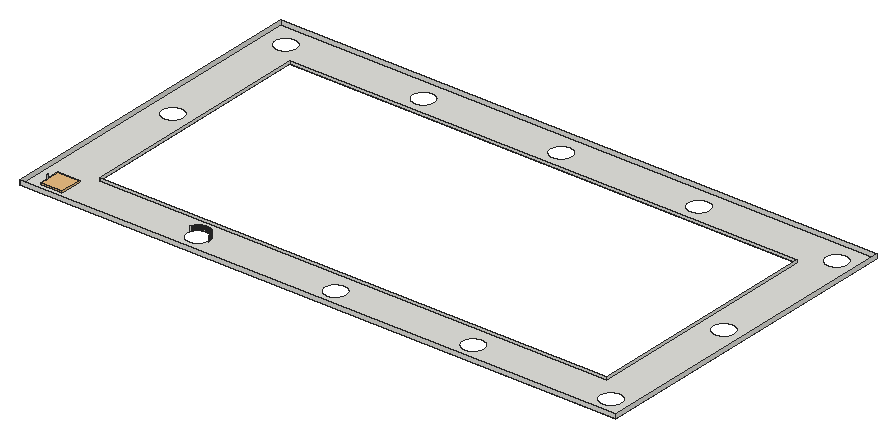
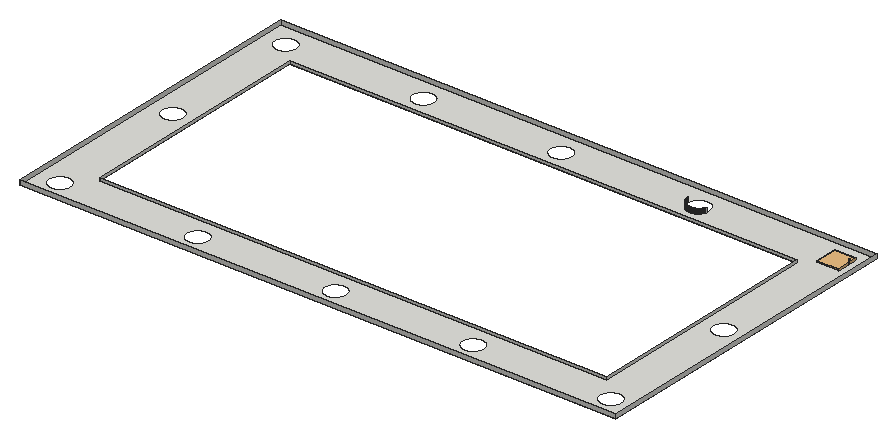
# SketchUp Ruby script. Lengths in inches.
U = 1.inch
M = Sketchup.active_model
def pt(a) = Geom::Point3d.new(a.map { |v| v * U })
def face(e, loops, mat)
  f = e.add_face(loops[0].map { |a| pt(a) })
  loops[1..].each { |l| e.add_face(l.map { |a| pt(a) }).erase! }
  f.material = f.back_material = mat if mat
  f
end
# faces: each face lists its corners as indices into pts; further lists are holes
def faces(e, pts, list, mat = nil) = list.each { |f| face(e, (f[0].is_a?(Array) ? f : [f]).map { |l| l.map { |i| pts[i] } }, mat) }
# xy, xz, yz: faces in a plane at the given z, y or x. An outline is a flat list of corners, or four numbers for a rectangle; further outlines are holes
def ring(l) = l.size == 4 ? [[l[0], l[1]], [l[2], l[1]], [l[2], l[3]], [l[0], l[3]]] : l.each_slice(2).to_a
def flat(e, list, mat, &to3) = list.each { |f| face(e, (f[0].is_a?(Array) ? f : [f]).map { |l| ring(l).map { |u, v| to3.(u, v) } }, mat) }
def xy(e, z, list, mat = nil) = flat(e, list, mat) { |x, y| [x, y, z] }
def xz(e, y, list, mat = nil) = flat(e, list, mat) { |x, z| [x, y, z] }
def yz(e, x, list, mat = nil) = flat(e, list, mat) { |y, z| [x, y, z] }
def lines(e, pts, list) = list.each { |a, b| e.add_line(pt(pts[a]), pt(pts[b])) }
# prism: a flat outline (further loops are holes) pulled along v
def prism(e, loops, v, mat = nil)
  f = face(e, loops, mat); d = Geom::Vector3d.new(v.map { |x| x * U })
  f.pushpull(f.normal.samedirection?(d) ? d.length : -d.length)
end
def box(e, o, s, mat = nil) = prism(e, [[o, [o[0] + s[0], o[1], o[2]], [o[0] + s[0], o[1] + s[1], o[2]], [o[0], o[1] + s[1], o[2]]]], [0, 0, s[2]], mat)
def at(x, y, z, deg = 0) = Geom::Transformation.translation(pt([x, y, z])) * Geom::Transformation.rotation(ORIGIN, Z_AXIS, deg.degrees)
def axes(o, x, y, z) = Geom::Transformation.new([*x, 0, *y, 0, *z, 0, *pt(o).to_a, 1])
def part(name) = M.definitions.add(name)
# library, detail: a bought-in or finely detailed component or shape, given as its bounding box
def library(name, o, s) = part(name).tap { |d| box(d.entities, o, s) }
def detail(e, o, s) = box(e.add_group.entities, o, s)
def put(e, d, t, mat = nil) = e.add_instance(d, t).tap { |i| i.material = mat if mat }
def group(e, t, mat = nil) = e.add_group.tap { |g| g.transformation = t; g.material = mat if mat }.entities
root = M.entities
c1 = library("plafonjera p5",[102.27,51.27,12.6],[3.93,3.93,0.39])
xy(root,231.53,[[[57.99,28,382.75,206],[81.99,52,358.75,182],[370.5625,188,370.9375,188,371.31,188.03,371.6875,188.07,372.06,188.14,372.42,188.24,372.78,188.35,373.13,188.49,373.47,188.65,373.8,188.84,374.12,189.04,374.43,189.26,374.72,189.5,374.99,189.76,375.25,190.03,375.49,190.32,375.71,190.63,375.91,190.95,376.1,191.28,376.26,191.62,376.4,191.97,376.51,192.33,376.61,192.69,376.68,193.0625,376.72,193.44,376.75,193.8125,376.75,194.1875,376.72,194.56,376.68,194.9375,376.61,195.31,376.51,195.67,376.4,196.03,376.26,196.38,376.1,196.72,375.91,197.05,375.71,197.37,375.49,197.68,375.25,197.97,374.99,198.24,374.72,198.5,374.43,198.74,374.12,198.96,373.8,199.16,373.47,199.35,373.13,199.51,372.78,199.65,372.42,199.76,372.06,199.86,371.6875,199.93,371.31,199.97,370.9375,200,370.5625,200,370.19,199.97,369.8125,199.93,369.44,199.86,369.08,199.76,368.72,199.65,368.37,199.51,368.03,199.35,367.7,199.16,367.38,198.96,367.07,198.74,366.78,198.5,366.51,198.24,366.25,197.97,366.01,197.68,365.79,197.37,365.59,197.05,365.4,196.72,365.24,196.38,365.1,196.03,364.99,195.67,364.89,195.31,364.82,194.9375,364.78,194.56,364.75,194.1875,364.75,193.8125,364.78,193.44,364.82,193.0625,364.89,192.69,364.99,192.33,365.1,191.97,365.24,191.62,365.4,191.28,365.59,190.95,365.79,190.63,366.01,190.32,366.25,190.03,366.51,189.76,366.78,189.5,367.07,189.26,367.38,189.04,367.7,188.84,368.03,188.65,368.37,188.49,368.72,188.35,369.08,188.24,369.44,188.14,369.8125,188.07,370.19,188.03],[220.18,188,220.56,188,220.94,188.03,221.31,188.07,221.68,188.14,222.04,188.24,222.4,188.35,222.75,188.49,223.09,188.65,223.43,188.84,223.74,189.04,224.05,189.26,224.34,189.5,224.61,189.76,224.87,190.03,225.11,190.32,225.33,190.63,225.54,190.95,225.72,191.28,225.88,191.62,226.02,191.97,226.13,192.33,226.23,192.69,226.3,193.0625,226.34,193.44,226.37,193.8125,226.37,194.1875,226.34,194.56,226.3,194.9375,226.23,195.31,226.13,195.67,226.02,196.03,225.88,196.38,225.72,196.72,225.54,197.05,225.33,197.37,225.11,197.68,224.87,197.97,224.61,198.24,224.34,198.5,224.05,198.74,223.74,198.96,223.43,199.16,223.09,199.35,222.75,199.51,222.4,199.65,222.04,199.76,221.68,199.86,221.31,199.93,220.94,199.97,220.56,200,220.18,200,219.81,199.97,219.43,199.93,219.0625,199.86,218.7,199.76,218.34,199.65,217.99,199.51,217.65,199.35,217.32,199.16,217,198.96,216.69,198.74,216.4,198.5,216.13,198.24,215.87,197.97,215.63,197.68,215.41,197.37,215.21,197.05,215.02,196.72,214.86,196.38,214.73,196.03,214.61,195.67,214.52,195.31,214.44,194.9375,214.4,194.56,214.375,194.1875,214.375,193.8125,214.4,193.44,214.44,193.0625,214.52,192.69,214.61,192.33,214.73,191.97,214.86,191.62,215.02,191.28,215.21,190.95,215.41,190.63,215.63,190.32,215.87,190.03,216.13,189.76,216.4,189.5,216.69,189.26,217,189.04,217.32,188.84,217.65,188.65,217.99,188.49,218.34,188.35,218.7,188.24,219.0625,188.14,219.43,188.07,219.81,188.03],[295.37,188,295.75,188,296.125,188.03,296.5,188.07,296.87,188.14,297.23,188.24,297.59,188.35,297.94,188.49,298.28,188.65,298.61,188.84,298.93,189.04,299.24,189.26,299.53,189.5,299.8,189.76,300.0625,190.03,300.3,190.32,300.52,190.63,300.72,190.95,300.91,191.28,301.07,191.62,301.21,191.97,301.32,192.33,301.42,192.69,301.49,193.0625,301.53,193.44,301.56,193.8125,301.56,194.1875,301.53,194.56,301.49,194.9375,301.42,195.31,301.32,195.67,301.21,196.03,301.07,196.38,300.91,196.72,300.72,197.05,300.52,197.37,300.3,197.68,300.0625,197.97,299.8,198.24,299.53,198.5,299.24,198.74,298.93,198.96,298.61,199.16,298.28,199.35,297.94,199.51,297.59,199.65,297.23,199.76,296.87,199.86,296.5,199.93,296.125,199.97,295.75,200,295.37,200,295,199.97,294.62,199.93,294.25,199.86,293.89,199.76,293.53,199.65,293.18,199.51,292.84,199.35,292.51,199.16,292.1875,198.96,291.88,198.74,291.59,198.5,291.32,198.24,291.06,197.97,290.82,197.68,290.6,197.37,290.4,197.05,290.21,196.72,290.05,196.38,289.92,196.03,289.8,195.67,289.7,195.31,289.63,194.9375,289.59,194.56,289.5625,194.1875,289.5625,193.8125,289.59,193.44,289.63,193.0625,289.7,192.69,289.8,192.33,289.92,191.97,290.05,191.62,290.21,191.28,290.4,190.95,290.6,190.63,290.82,190.32,291.06,190.03,291.32,189.76,291.59,189.5,291.88,189.26,292.1875,189.04,292.51,188.84,292.84,188.65,293.18,188.49,293.53,188.35,293.89,188.24,294.25,188.14,294.62,188.07,295,188.03],[370.5625,111,370.9375,111,371.31,111.03,371.6875,111.07,372.06,111.14,372.42,111.24,372.78,111.35,373.13,111.49,373.47,111.65,373.8,111.84,374.12,112.04,374.43,112.26,374.72,112.5,374.99,112.76,375.25,113.03,375.49,113.32,375.71,113.63,375.91,113.95,376.1,114.28,376.26,114.62,376.4,114.97,376.51,115.33,376.61,115.69,376.68,116.0625,376.72,116.44,376.75,116.8125,376.75,117.1875,376.72,117.56,376.68,117.9375,376.61,118.31,376.51,118.67,376.4,119.03,376.26,119.38,376.1,119.72,375.91,120.05,375.71,120.37,375.49,120.68,375.25,120.97,374.99,121.24,374.72,121.5,374.43,121.74,374.12,121.96,373.8,122.16,373.47,122.35,373.13,122.51,372.78,122.65,372.42,122.76,372.06,122.86,371.6875,122.93,371.31,122.97,370.9375,123,370.5625,123,370.19,122.97,369.8125,122.93,369.44,122.86,369.08,122.76,368.72,122.65,368.37,122.51,368.03,122.35,367.7,122.16,367.38,121.96,367.07,121.74,366.78,121.5,366.51,121.24,366.25,120.97,366.01,120.68,365.79,120.37,365.59,120.05,365.4,119.72,365.24,119.38,365.1,119.03,364.99,118.67,364.89,118.31,364.82,117.9375,364.78,117.56,364.75,117.1875,364.75,116.8125,364.78,116.44,364.82,116.0625,364.89,115.69,364.99,115.33,365.1,114.97,365.24,114.62,365.4,114.28,365.59,113.95,365.79,113.63,366.01,113.32,366.25,113.03,366.51,112.76,366.78,112.5,367.07,112.26,367.38,112.04,367.7,111.84,368.03,111.65,368.37,111.49,368.72,111.35,369.08,111.24,369.44,111.14,369.8125,111.07,370.19,111.03],[69.8,34,70.18,34,70.56,34.03,70.93,34.07,71.3,34.14,71.67,34.24,72.02,34.35,72.375,34.49,72.72,34.65,73.05,34.84,73.36,35.04,73.67,35.26,73.96,35.5,74.23,35.76,74.49,36.03,74.73,36.32,74.95,36.63,75.16,36.95,75.34,37.28,75.5,37.62,75.64,37.97,75.75,38.33,75.85,38.69,75.92,39.0625,75.96,39.44,75.99,39.8125,75.99,40.1875,75.96,40.56,75.92,40.9375,75.85,41.31,75.75,41.67,75.64,42.03,75.5,42.38,75.34,42.72,75.16,43.05,74.95,43.37,74.73,43.68,74.49,43.97,74.23,44.24,73.96,44.5,73.67,44.74,73.36,44.96,73.05,45.16,72.72,45.35,72.375,45.51,72.02,45.65,71.67,45.76,71.3,45.86,70.93,45.93,70.56,45.97,70.18,46,69.8,46,69.43,45.97,69.05,45.93,68.68,45.86,68.32,45.76,67.96,45.65,67.61,45.51,67.27,45.35,66.9375,45.16,66.62,44.96,66.3125,44.74,66.02,44.5,65.75,44.24,65.49,43.97,65.25,43.68,65.03,43.37,64.83,43.05,64.65,42.72,64.48,42.38,64.35,42.03,64.23,41.67,64.14,41.31,64.07,40.9375,64.02,40.56,63.99,40.1875,63.99,39.8125,64.02,39.44,64.07,39.0625,64.14,38.69,64.23,38.33,64.35,37.97,64.48,37.62,64.65,37.28,64.83,36.95,65.03,36.63,65.25,36.32,65.49,36.03,65.75,35.76,66.02,35.5,66.3125,35.26,66.62,35.04,66.9375,34.84,67.27,34.65,67.61,34.49,67.96,34.35,68.32,34.24,68.68,34.14,69.05,34.07,69.43,34.03],[69.8,111,70.18,111,70.56,111.03,70.93,111.07,71.3,111.14,71.67,111.24,72.02,111.35,72.375,111.49,72.72,111.65,73.05,111.84,73.36,112.04,73.67,112.26,73.96,112.5,74.23,112.76,74.49,113.03,74.73,113.32,74.95,113.63,75.16,113.95,75.34,114.28,75.5,114.62,75.64,114.97,75.75,115.33,75.85,115.69,75.92,116.0625,75.96,116.44,75.99,116.8125,75.99,117.1875,75.96,117.56,75.92,117.9375,75.85,118.31,75.75,118.67,75.64,119.03,75.5,119.38,75.34,119.72,75.16,120.05,74.95,120.37,74.73,120.68,74.49,120.97,74.23,121.24,73.96,121.5,73.67,121.74,73.36,121.96,73.05,122.16,72.72,122.35,72.375,122.51,72.02,122.65,71.67,122.76,71.3,122.86,70.93,122.93,70.56,122.97,70.18,123,69.8,123,69.43,122.97,69.05,122.93,68.68,122.86,68.32,122.76,67.96,122.65,67.61,122.51,67.27,122.35,66.9375,122.16,66.62,121.96,66.3125,121.74,66.02,121.5,65.75,121.24,65.49,120.97,65.25,120.68,65.03,120.37,64.83,120.05,64.65,119.72,64.48,119.38,64.35,119.03,64.23,118.67,64.14,118.31,64.07,117.9375,64.02,117.56,63.99,117.1875,63.99,116.8125,64.02,116.44,64.07,116.0625,64.14,115.69,64.23,115.33,64.35,114.97,64.48,114.62,64.65,114.28,64.83,113.95,65.03,113.63,65.25,113.32,65.49,113.03,65.75,112.76,66.02,112.5,66.3125,112.26,66.62,112.04,66.9375,111.84,67.27,111.65,67.61,111.49,67.96,111.35,68.32,111.24,68.68,111.14,69.05,111.07,69.43,111.03],[144.99,34,145.37,34,145.75,34.03,146.12,34.07,146.49,34.14,146.86,34.24,147.21,34.35,147.5625,34.49,147.91,34.65,148.24,34.84,148.55,35.04,148.86,35.26,149.15,35.5,149.42,35.76,149.68,36.03,149.92,36.32,150.14,36.63,150.35,36.95,150.53,37.28,150.6875,37.62,150.83,37.97,150.94,38.33,151.04,38.69,151.11,39.0625,151.15,39.44,151.18,39.8125,151.18,40.1875,151.15,40.56,151.11,40.9375,151.04,41.31,150.94,41.67,150.83,42.03,150.6875,42.38,150.53,42.72,150.35,43.05,150.14,43.37,149.92,43.68,149.68,43.97,149.42,44.24,149.15,44.5,148.86,44.74,148.55,44.96,148.24,45.16,147.91,45.35,147.5625,45.51,147.21,45.65,146.86,45.76,146.49,45.86,146.12,45.93,145.75,45.97,145.37,46,144.99,46,144.62,45.97,144.24,45.93,143.87,45.86,143.51,45.76,143.15,45.65,142.8,45.51,142.46,45.35,142.125,45.16,141.81,44.96,141.5,44.74,141.21,44.5,140.9375,44.24,140.68,43.97,140.44,43.68,140.22,43.37,140.02,43.05,139.84,42.72,139.67,42.38,139.54,42.03,139.42,41.67,139.33,41.31,139.26,40.9375,139.21,40.56,139.18,40.1875,139.18,39.8125,139.21,39.44,139.26,39.0625,139.33,38.69,139.42,38.33,139.54,37.97,139.67,37.62,139.84,37.28,140.02,36.95,140.22,36.63,140.44,36.32,140.68,36.03,140.9375,35.76,141.21,35.5,141.5,35.26,141.81,35.04,142.125,34.84,142.46,34.65,142.8,34.49,143.15,34.35,143.51,34.24,143.87,34.14,144.24,34.07,144.62,34.03],[144.99,188,145.37,188,145.75,188.03,146.12,188.07,146.49,188.14,146.86,188.24,147.21,188.35,147.5625,188.49,147.91,188.65,148.24,188.84,148.55,189.04,148.86,189.26,149.15,189.5,149.42,189.76,149.68,190.03,149.92,190.32,150.14,190.63,150.35,190.95,150.53,191.28,150.6875,191.62,150.83,191.97,150.94,192.33,151.04,192.69,151.11,193.0625,151.15,193.44,151.18,193.8125,151.18,194.1875,151.15,194.56,151.11,194.9375,151.04,195.31,150.94,195.67,150.83,196.03,150.6875,196.38,150.53,196.72,150.35,197.05,150.14,197.37,149.92,197.68,149.68,197.97,149.42,198.24,149.15,198.5,148.86,198.74,148.55,198.96,148.24,199.16,147.91,199.35,147.5625,199.51,147.21,199.65,146.86,199.76,146.49,199.86,146.12,199.93,145.75,199.97,145.37,200,144.99,200,144.62,199.97,144.24,199.93,143.87,199.86,143.51,199.76,143.15,199.65,142.8,199.51,142.46,199.35,142.125,199.16,141.81,198.96,141.5,198.74,141.21,198.5,140.9375,198.24,140.68,197.97,140.44,197.68,140.22,197.37,140.02,197.05,139.84,196.72,139.67,196.38,139.54,196.03,139.42,195.67,139.33,195.31,139.26,194.9375,139.21,194.56,139.18,194.1875,139.18,193.8125,139.21,193.44,139.26,193.0625,139.33,192.69,139.42,192.33,139.54,191.97,139.67,191.62,139.84,191.28,140.02,190.95,140.22,190.63,140.44,190.32,140.68,190.03,140.9375,189.76,141.21,189.5,141.5,189.26,141.81,189.04,142.125,188.84,142.46,188.65,142.8,188.49,143.15,188.35,143.51,188.24,143.87,188.14,144.24,188.07,144.62,188.03],[370.5625,34,370.9375,34,371.31,34.03,371.6875,34.07,372.06,34.14,372.42,34.24,372.78,34.35,373.13,34.49,373.47,34.65,373.8,34.84,374.12,35.04,374.43,35.26,374.72,35.5,374.99,35.76,375.25,36.03,375.49,36.32,375.71,36.63,375.91,36.95,376.1,37.28,376.26,37.62,376.4,37.97,376.51,38.33,376.61,38.69,376.68,39.0625,376.72,39.44,376.75,39.8125,376.75,40.1875,376.72,40.56,376.68,40.9375,376.61,41.31,376.51,41.67,376.4,42.03,376.26,42.38,376.1,42.72,375.91,43.05,375.71,43.37,375.49,43.68,375.25,43.97,374.99,44.24,374.72,44.5,374.43,44.74,374.12,44.96,373.8,45.16,373.47,45.35,373.13,45.51,372.78,45.65,372.42,45.76,372.06,45.86,371.6875,45.93,371.31,45.97,370.9375,46,370.5625,46,370.19,45.97,369.8125,45.93,369.44,45.86,369.08,45.76,368.72,45.65,368.37,45.51,368.03,45.35,367.7,45.16,367.38,44.96,367.07,44.74,366.78,44.5,366.51,44.24,366.25,43.97,366.01,43.68,365.79,43.37,365.59,43.05,365.4,42.72,365.24,42.38,365.1,42.03,364.99,41.67,364.89,41.31,364.82,40.9375,364.78,40.56,364.75,40.1875,364.75,39.8125,364.78,39.44,364.82,39.0625,364.89,38.69,364.99,38.33,365.1,37.97,365.24,37.62,365.4,37.28,365.59,36.95,365.79,36.63,366.01,36.32,366.25,36.03,366.51,35.76,366.78,35.5,367.07,35.26,367.38,35.04,367.7,34.84,368.03,34.65,368.37,34.49,368.72,34.35,369.08,34.24,369.44,34.14,369.8125,34.07,370.19,34.03],[220.18,34,220.56,34,220.94,34.03,221.31,34.07,221.68,34.14,222.04,34.24,222.4,34.35,222.75,34.49,223.09,34.65,223.43,34.84,223.74,35.04,224.05,35.26,224.34,35.5,224.61,35.76,224.87,36.03,225.11,36.32,225.33,36.63,225.54,36.95,225.72,37.28,225.88,37.62,226.02,37.97,226.13,38.33,226.23,38.69,226.3,39.0625,226.34,39.44,226.37,39.8125,226.37,40.1875,226.34,40.56,226.3,40.9375,226.23,41.31,226.13,41.67,226.02,42.03,225.88,42.38,225.72,42.72,225.54,43.05,225.33,43.37,225.11,43.68,224.87,43.97,224.61,44.24,224.34,44.5,224.05,44.74,223.74,44.96,223.43,45.16,223.09,45.35,222.75,45.51,222.4,45.65,222.04,45.76,221.68,45.86,221.31,45.93,220.94,45.97,220.56,46,220.18,46,219.81,45.97,219.43,45.93,219.0625,45.86,218.7,45.76,218.34,45.65,217.99,45.51,217.65,45.35,217.32,45.16,217,44.96,216.69,44.74,216.4,44.5,216.13,44.24,215.87,43.97,215.63,43.68,215.41,43.37,215.21,43.05,215.02,42.72,214.86,42.38,214.73,42.03,214.61,41.67,214.52,41.31,214.44,40.9375,214.4,40.56,214.375,40.1875,214.375,39.8125,214.4,39.44,214.44,39.0625,214.52,38.69,214.61,38.33,214.73,37.97,214.86,37.62,215.02,37.28,215.21,36.95,215.41,36.63,215.63,36.32,215.87,36.03,216.13,35.76,216.4,35.5,216.69,35.26,217,35.04,217.32,34.84,217.65,34.65,217.99,34.49,218.34,34.35,218.7,34.24,219.0625,34.14,219.43,34.07,219.81,34.03],[295.37,34,295.75,34,296.125,34.03,296.5,34.07,296.87,34.14,297.23,34.24,297.59,34.35,297.94,34.49,298.28,34.65,298.61,34.84,298.93,35.04,299.24,35.26,299.53,35.5,299.8,35.76,300.0625,36.03,300.3,36.32,300.52,36.63,300.72,36.95,300.91,37.28,301.07,37.62,301.21,37.97,301.32,38.33,301.42,38.69,301.49,39.0625,301.53,39.44,301.56,39.8125,301.56,40.1875,301.53,40.56,301.49,40.9375,301.42,41.31,301.32,41.67,301.21,42.03,301.07,42.38,300.91,42.72,300.72,43.05,300.52,43.37,300.3,43.68,300.0625,43.97,299.8,44.24,299.53,44.5,299.24,44.74,298.93,44.96,298.61,45.16,298.28,45.35,297.94,45.51,297.59,45.65,297.23,45.76,296.87,45.86,296.5,45.93,296.125,45.97,295.75,46,295.37,46,295,45.97,294.62,45.93,294.25,45.86,293.89,45.76,293.53,45.65,293.18,45.51,292.84,45.35,292.51,45.16,292.1875,44.96,291.88,44.74,291.59,44.5,291.32,44.24,291.06,43.97,290.82,43.68,290.6,43.37,290.4,43.05,290.21,42.72,290.05,42.38,289.92,42.03,289.8,41.67,289.7,41.31,289.63,40.9375,289.59,40.56,289.5625,40.1875,289.5625,39.8125,289.59,39.44,289.63,39.0625,289.7,38.69,289.8,38.33,289.92,37.97,290.05,37.62,290.21,37.28,290.4,36.95,290.6,36.63,290.82,36.32,291.06,36.03,291.32,35.76,291.59,35.5,291.88,35.26,292.1875,35.04,292.51,34.84,292.84,34.65,293.18,34.49,293.53,34.35,293.89,34.24,294.25,34.14,294.62,34.07,295,34.03],[69.8,188,70.18,188,70.56,188.03,70.93,188.07,71.3,188.14,71.67,188.24,72.02,188.35,72.375,188.49,72.72,188.65,73.05,188.84,73.36,189.04,73.67,189.26,73.96,189.5,74.23,189.76,74.49,190.03,74.73,190.32,74.95,190.63,75.16,190.95,75.34,191.28,75.5,191.62,75.64,191.97,75.75,192.33,75.85,192.69,75.92,193.0625,75.96,193.44,75.99,193.8125,75.99,194.1875,75.96,194.56,75.92,194.9375,75.85,195.31,75.75,195.67,75.64,196.03,75.5,196.38,75.34,196.72,75.16,197.05,74.95,197.37,74.73,197.68,74.49,197.97,74.23,198.24,73.96,198.5,73.67,198.74,73.36,198.96,73.05,199.16,72.72,199.35,72.375,199.51,72.02,199.65,71.67,199.76,71.3,199.86,70.93,199.93,70.56,199.97,70.18,200,69.8,200,69.43,199.97,69.05,199.93,68.68,199.86,68.32,199.76,67.96,199.65,67.61,199.51,67.27,199.35,66.9375,199.16,66.62,198.96,66.3125,198.74,66.02,198.5,65.75,198.24,65.49,197.97,65.25,197.68,65.03,197.37,64.83,197.05,64.65,196.72,64.48,196.38,64.35,196.03,64.23,195.67,64.14,195.31,64.07,194.9375,64.02,194.56,63.99,194.1875,63.99,193.8125,64.02,193.44,64.07,193.0625,64.14,192.69,64.23,192.33,64.35,191.97,64.48,191.62,64.65,191.28,64.83,190.95,65.03,190.63,65.25,190.32,65.49,190.03,65.75,189.76,66.02,189.5,66.3125,189.26,66.62,189.04,66.9375,188.84,67.27,188.65,67.61,188.49,67.96,188.35,68.32,188.24,68.68,188.14,69.05,188.07,69.43,188.03]]])
xz(root,28,[[57.99,231.53,382.75,234]])
xz(root,46,[[144.99,231.53,145.37,234]])
xz(root,52,[[81.99,231.53,358.75,233]])
xz(root,182,[[81.99,231.53,358.75,233]])
xz(root,206,[[57.99,231.53,382.75,234]])
yz(root,57.99,[[28,231.53,206,234]])
yz(root,81.99,[[52,231.53,182,233]])
yz(root,151.18,[[39.8125,231.53,40.1875,234]])
yz(root,358.75,[[52,231.53,182,233]])
yz(root,382.75,[[28,231.53,206,234]])
p = [[64.14,38.69,231.53],[64.07,39.0625,231.53],[64.07,39.0625,234],[64.14,38.69,234],[64.02,39.44,231.53],[64.02,39.44,234],
  [151.15,40.56,231.53],[151.18,40.1875,231.53],[151.18,40.1875,234],[151.15,40.56,234],[151.11,40.9375,231.53],[151.11,40.9375,234],
  [151.04,41.31,231.53],[151.04,41.31,234],[150.94,41.67,231.53],[150.94,41.67,234],[150.83,42.03,231.53],[150.83,42.03,234],
  [139.54,42.03,231.53],[139.67,42.38,231.53],[139.67,42.38,234],[139.54,42.03,234],[150.6875,42.38,231.53],[150.6875,42.38,234],
  [139.84,42.72,231.53],[139.84,42.72,234],[150.53,42.72,231.53],[150.53,42.72,234],[140.02,43.05,231.53],[140.02,43.05,234],
  [150.35,43.05,231.53],[150.35,43.05,234],[140.22,43.37,231.53],[140.22,43.37,234],[150.14,43.37,231.53],[150.14,43.37,234],
  [140.44,43.68,231.53],[140.44,43.68,234],[149.92,43.68,231.53],[149.92,43.68,234],[140.68,43.97,231.53],[140.68,43.97,234],
  [149.68,43.97,231.53],[149.68,43.97,234],[140.9375,44.24,231.53],[140.9375,44.24,234],[149.42,44.24,231.53],[149.42,44.24,234],
  [141.21,44.5,231.53],[141.21,44.5,234],[149.15,44.5,231.53],[149.15,44.5,234],[141.5,44.74,231.53],[141.5,44.74,234],
  [148.86,44.74,231.53],[148.86,44.74,234],[141.81,44.96,231.53],[141.81,44.96,234],[148.55,44.96,231.53],[148.55,44.96,234],
  [142.125,45.16,231.53],[142.125,45.16,234],[148.24,45.16,231.53],[148.24,45.16,234],[142.46,45.35,231.53],[142.46,45.35,234],
  [147.91,45.35,231.53],[147.91,45.35,234],[142.8,45.51,231.53],[142.8,45.51,234],[147.5625,45.51,231.53],[147.5625,45.51,234],
  [143.15,45.65,231.53],[143.15,45.65,234],[147.21,45.65,231.53],[147.21,45.65,234],[143.51,45.76,231.53],[143.51,45.76,234],
  [146.86,45.76,231.53],[146.86,45.76,234],[143.87,45.86,231.53],[143.87,45.86,234],[146.49,45.86,231.53],[146.49,45.86,234],
  [144.24,45.93,231.53],[144.24,45.93,234],[144.62,45.97,231.53],[144.62,45.97,234],[145.75,45.97,231.53],[146.12,45.93,231.53],
  [146.12,45.93,234],[145.75,45.97,234],[144.99,46,231.53],[144.99,46,234],[145.37,46,231.53],[145.37,46,234]]
faces(root,p,[[0,1,2,3],[1,4,5,2],[6,7,8,9],[10,6,9,11],[12,10,11,13],[14,12,13,15],[16,14,15,17],[18,19,20,21],
  [22,16,17,23],[19,24,25,20],[26,22,23,27],[24,28,29,25],[30,26,27,31],[28,32,33,29],[34,30,31,35],[32,36,37,33],
  [38,34,35,39],[36,40,41,37],[42,38,39,43],[40,44,45,41],[46,42,43,47],[44,48,49,45],[50,46,47,51],[48,52,53,49],
  [54,50,51,55],[52,56,57,53],[58,54,55,59],[56,60,61,57],[62,58,59,63],[60,64,65,61],[66,62,63,67],[64,68,69,65],
  [70,66,67,71],[68,72,73,69],[74,70,71,75],[72,76,77,73],[78,74,75,79],[76,80,81,77],[82,78,79,83],[80,84,85,81],
  [84,86,87,85],[88,89,90,91],[89,82,83,90],[86,92,93,87],[94,88,91,95]])
put(root,c1,axes([-242.72,-119.71,193.26],[3,0,0],[0,3,0],[0,0,3]))
